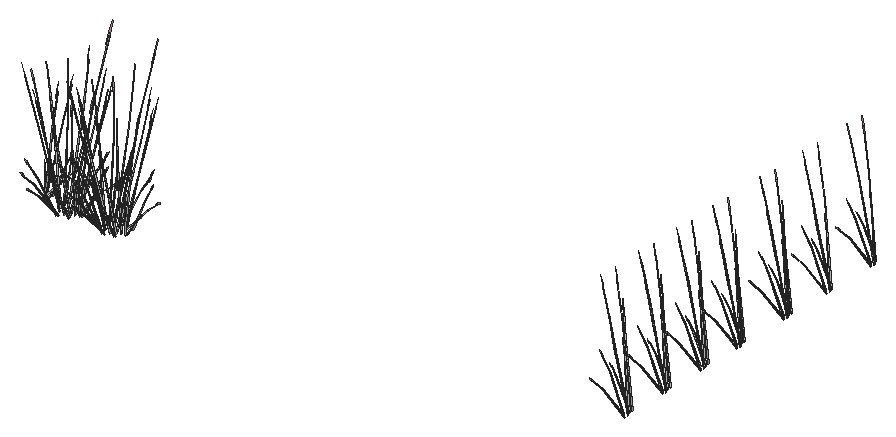
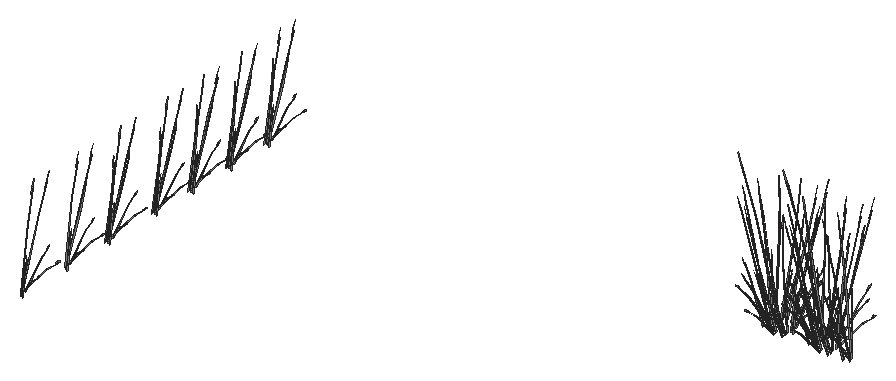
# SketchUp Ruby script. Lengths in inches.
U = 1.inch
M = Sketchup.active_model
def pt(a) = Geom::Point3d.new(a.map { |v| v * U })
def face(e, loops, mat)
  f = e.add_face(loops[0].map { |a| pt(a) })
  loops[1..].each { |l| e.add_face(l.map { |a| pt(a) }).erase! }
  f.material = f.back_material = mat if mat
  f
end
# faces: each face lists its corners as indices into pts; further lists are holes
def faces(e, pts, list, mat = nil) = list.each { |f| face(e, (f[0].is_a?(Array) ? f : [f]).map { |l| l.map { |i| pts[i] } }, mat) }
# xy, xz, yz: faces in a plane at the given z, y or x. An outline is a flat list of corners, or four numbers for a rectangle; further outlines are holes
def ring(l) = l.size == 4 ? [[l[0], l[1]], [l[2], l[1]], [l[2], l[3]], [l[0], l[3]]] : l.each_slice(2).to_a
def flat(e, list, mat, &to3) = list.each { |f| face(e, (f[0].is_a?(Array) ? f : [f]).map { |l| ring(l).map { |u, v| to3.(u, v) } }, mat) }
def xy(e, z, list, mat = nil) = flat(e, list, mat) { |x, y| [x, y, z] }
def xz(e, y, list, mat = nil) = flat(e, list, mat) { |x, z| [x, y, z] }
def yz(e, x, list, mat = nil) = flat(e, list, mat) { |y, z| [x, y, z] }
def lines(e, pts, list) = list.each { |a, b| e.add_line(pt(pts[a]), pt(pts[b])) }
# prism: a flat outline (further loops are holes) pulled along v
def prism(e, loops, v, mat = nil)
  f = face(e, loops, mat); d = Geom::Vector3d.new(v.map { |x| x * U })
  f.pushpull(f.normal.samedirection?(d) ? d.length : -d.length)
end
def box(e, o, s, mat = nil) = prism(e, [[o, [o[0] + s[0], o[1], o[2]], [o[0] + s[0], o[1] + s[1], o[2]], [o[0], o[1] + s[1], o[2]]]], [0, 0, s[2]], mat)
def at(x, y, z, deg = 0) = Geom::Transformation.translation(pt([x, y, z])) * Geom::Transformation.rotation(ORIGIN, Z_AXIS, deg.degrees)
def axes(o, x, y, z) = Geom::Transformation.new([*x, 0, *y, 0, *z, 0, *pt(o).to_a, 1])
def part(name) = M.definitions.add(name)
# library, detail: a bought-in or finely detailed component or shape, given as its bounding box
def library(name, o, s) = part(name).tap { |d| box(d.entities, o, s) }
def detail(e, o, s) = box(e.add_group.entities, o, s)
def put(e, d, t, mat = nil) = e.add_instance(d, t).tap { |i| i.material = mat if mat }
def group(e, t, mat = nil) = e.add_group.tap { |g| g.transformation = t; g.material = mat if mat }.entities
root = M.entities
M.materials.add("LightPink_Translucent").color = [144, 107, 117]
M.materials["LightPink_Translucent"].alpha = 0.75
M.materials.add("[_0053_Ivory_]").color = [200, 200, 200]
c1 = part("blade")
p = [[2.15,0.21,22],[0,0.17,0],[0.09,0.45,0],[2.18,0.31,22],[2.29,0.31,22],[0.38,0.45,0],
  [2.48,0.24,33],[2.49,0.24,33],[2.48,0.22,33]]
faces(c1.entities,p,[[0,1,2,3],[4,5,2,3],[6,3,4,7],[8,0,3,6]])
c2 = part("seeds")
p = [[0.3,-0.1,1.38],[-0.01,-0.03,1.59],[-0.01,-0.03,0.03],[0.14,-0.07,-0.07],[0.29,-0.03,3],[0.15,0.01,3.11]]
faces(c2.entities,p,[[0,1,2,3],[1,0,4,5]],"LightPink_Translucent")
c3 = part("blade with seeds")
put(c3.entities,c1,at(0,0,0))
put(c3.entities,c2,axes([2.4,0.25,30.99],[1.5799,-0.05474,1.17369],[-0.12525,1.92788,0.29478],[-0.07173,-0.02425,1.56792]))
put(root,c3,axes([467.79,99.63,131.37],[-0.13068,-0.00444,1.74944],[-0.41604,0.44388,-0.27667],[-0.22198,-0.0907,0.14031]),"[_0053_Ivory_]")
put(root,c3,axes([467.45,101.92,131.6875],[0.30559,0.56943,-0.1216],[-0.54237,0.27983,-0.67495],[-0.22856,0.07513,1.02557]),"[_0053_Ivory_]")
put(root,c3,axes([468.14,100.74,131.6875],[-0.03252,0.63953,-0.1216],[-0.61574,-0.01748,-0.67495],[-0.23714,-0.04442,1.02557]),"[_0053_Ivory_]")
put(root,c3,axes([462.59,102.55,131.36],[-0.07933,-0.00478,1.77383],[-0.32942,-0.51175,-0.16761],[0.13229,-0.16826,0.31391]),"[_0053_Ivory_]")
put(root,c3,axes([466.83,104.72,131.37],[-0.0151,0.12444,1.74944],[0.42844,0.43292,-0.27667],[-0.11216,0.20472,0.14031]),"[_0053_Ivory_]")
put(root,c3,axes([469.34,99.81,132.08],[-0.40534,0.60286,-0.13619],[-0.58702,-0.34732,-0.75594],[-0.20405,-0.17032,1.14864]),"[_0053_Ivory_]")
put(root,c3,axes([460.55,105.23,131.6875],[0.03252,-0.63953,-0.1216],[0.61574,0.01748,-0.67495],[0.23714,0.04442,1.02557]),"[_0053_Ivory_]")
put(root,c3,axes([461.23,104.05,131.6875],[-0.30559,-0.56943,-0.1216],[0.54237,-0.27983,-0.67495],[0.22856,-0.07513,1.02557]),"[_0053_Ivory_]")
put(root,c3,axes([467.47,103.28,131.6875],[0.56181,0.34675,-0.1216],[-0.32367,0.50216,-0.67495],[-0.15873,0.17455,1.02557]),"[_0053_Ivory_]")
put(root,c3,axes([461.08,104.85,131.37],[0.13029,-0.01064,1.74944],[0.35737,-0.48855,-0.27667],[0.23175,0.06449,0.14031]),"[_0053_Ivory_]")
put(root,c3,axes([469.18,98.37,131.36],[-0.01133,0.07538,1.77383],[-0.55883,0.27355,-0.16761],[-0.16445,-0.13983,0.31391]),"[_0053_Ivory_]")
put(root,c3,axes([462.45,105.74,131.36],[-0.05492,-0.05505,1.77383],[0.12013,-0.59013,-0.16761],[0.21632,-0.0377,0.31391]),"[_0053_Ivory_]")
put(root,c3,axes([466.78,105.99,131.36],[0.0689,-0.03797,1.77383],[0.5695,0.25254,-0.16761],[-0.01338,0.21027,0.31391]),"[_0053_Ivory_]")
put(root,c3,axes([462.89,103.16,131.37],[0.08428,-0.09579,1.74944],[-0.10787,-0.58756,-0.27667],[0.21147,-0.1114,0.14031]),"[_0053_Ivory_]")
put(root,c3,axes([469.82,98.66,131.37],[-0.0929,-0.08817,1.74944],[-0.61994,0.0559,-0.27667],[-0.09894,-0.21089,0.14031]),"[_0053_Ivory_]")
put(root,c3,axes([468.2,104.4375,132.05],[0.6675,0.03116,-0.13498],[-0.01824,0.58993,-0.74919],[-0.04637,0.2272,1.13838]),"[_0053_Ivory_]")
put(root,c3,axes([470.76,100.02,131.6875],[-0.59433,0.29278,-0.1216],[-0.29207,-0.51964,-0.67495],[-0.07842,-0.21898,1.02557]),"[_0053_Ivory_]")
put(root,c3,axes([469.29,106.26,131.37],[0.07699,0.10127,1.74944],[0.6213,0.03978,-0.27667],[0.06248,0.22333,0.14031]),"[_0053_Ivory_]")
put(root,c3,axes([469.43,105.09,131.6875],[0.59433,-0.29278,-0.1216],[0.29207,0.51964,-0.67495],[0.07842,0.21898,1.02557]),"[_0053_Ivory_]")
put(root,c3,axes([472.47,99.29,131.36],[-0.06168,0.04803,1.77383],[-0.60432,-0.16205,-0.16761],[-0.02188,-0.20961,0.31391]),"[_0053_Ivory_]")
put(root,c3,axes([472,100.68,131.6875],[-0.6675,-0.03116,-0.1216],[0.01824,-0.58993,-0.67495],[0.04637,-0.2272,1.02557]),"[_0053_Ivory_]")
put(root,c3,axes([471.26,101.9,131.13],[-0.52482,-0.32674,1.38283],[0.55416,-0.50872,0.59665],[0.16933,0.30658,1.33663]),"[_0053_Ivory_]")
put(root,c3,axes([470.375,105.52,131.36],[0.0018,-0.07613,1.77383],[0.52048,-0.3359,-0.16761],[0.18079,0.11989,0.31391]),"[_0053_Ivory_]")
put(root,c3,axes([472.6,99.74,131.37],[-0.00586,-0.12516,1.74944],[-0.49517,-0.36172,-0.27667],[0.07656,-0.21927,0.14031]),"[_0053_Ivory_]")
put(root,c3,axes([470.85,105.07,131.6875],[0.36191,-0.53827,-0.1216],[0.52412,0.3101,-0.67495],[0.18219,0.15207,1.02557]),"[_0053_Ivory_]")
put(root,c3,axes([472.72,101.84,131.6875],[-0.56181,-0.34675,-0.1216],[0.32367,-0.50216,-0.67495],[0.15873,-0.17455,1.02557]),"[_0053_Ivory_]")
put(root,c3,axes([474.11,101.69,131.36],[-0.07933,-0.00478,1.77383],[-0.32942,-0.51175,-0.16761],[0.13229,-0.16826,0.31391]),"[_0053_Ivory_]")
put(root,c3,axes([472.06,104.38,131.6875],[0.03252,-0.63953,-0.1216],[0.61574,0.01748,-0.67495],[0.23714,0.04442,1.02557]),"[_0053_Ivory_]")
put(root,c3,axes([472.75,103.19,131.6875],[-0.30559,-0.56943,-0.1216],[0.54237,-0.27983,-0.67495],[0.22856,-0.07513,1.02557]),"[_0053_Ivory_]")
put(root,c3,axes([481.3,102.28,131.37],[-0.09918,0.08165,1.74944],[0.00844,0.59653,-0.27667],[-0.22734,0.07758,0.14031]),"[_0053_Ivory_]")
put(root,c3,axes([472.59,103.99,131.37],[0.13029,-0.01064,1.74944],[0.35737,-0.48855,-0.27667],[0.23175,0.06449,0.14031]),"[_0053_Ivory_]")
put(root,c3,axes([480.2,102.88,131.36],[0.07751,0.01687,1.77383],[0.23978,0.55562,-0.16761],[-0.15867,0.14583,0.31391]),"[_0053_Ivory_]")
put(root,c3,axes([481.77,99.8,131.36],[0.04503,0.06276,1.77383],[-0.21706,0.56413,-0.16761],[-0.21983,0.00408,0.31391]),"[_0053_Ivory_]")
put(root,c3,axes([473.96,104.89,131.36],[-0.05492,-0.05505,1.77383],[0.12013,-0.59013,-0.16761],[0.21632,-0.0377,0.31391]),"[_0053_Ivory_]")
put(root,c3,axes([482.28,99.42,131.37],[-0.13068,-0.00444,1.74944],[-0.41604,0.44388,-0.27667],[-0.22198,-0.0907,0.14031]),"[_0053_Ivory_]")
put(root,c3,axes([481.94,101.71,131.6875],[0.30559,0.56943,-0.1216],[-0.54237,0.27983,-0.67495],[-0.22856,0.07513,1.02557]),"[_0053_Ivory_]")
put(root,c3,axes([482.63,100.53,131.6875],[-0.03252,0.63953,-0.1216],[-0.61574,-0.01748,-0.67495],[-0.23714,-0.04442,1.02557]),"[_0053_Ivory_]")
put(root,c3,axes([474.41,102.3,131.37],[0.08428,-0.09579,1.74944],[-0.10787,-0.58756,-0.27667],[0.21147,-0.1114,0.14031]),"[_0053_Ivory_]")
put(root,c3,axes([481.32,104.51,131.37],[-0.0151,0.12444,1.74944],[0.42844,0.43292,-0.27667],[-0.11216,0.20472,0.14031]),"[_0053_Ivory_]")
put(root,c3,axes([483.83,99.6,132.08],[-0.40534,0.60286,-0.13619],[-0.58702,-0.34732,-0.75594],[-0.20405,-0.17032,1.14864]),"[_0053_Ivory_]")
put(root,c3,axes([481.97,103.07,131.6875],[0.56181,0.34675,-0.1216],[-0.32367,0.50216,-0.67495],[-0.15873,0.17455,1.02557]),"[_0053_Ivory_]")
put(root,c3,axes([483.67,98.16,131.36],[-0.01133,0.07538,1.77383],[-0.55883,0.27355,-0.16761],[-0.16445,-0.13983,0.31391]),"[_0053_Ivory_]")
put(root,c3,axes([481.27,105.78,131.36],[0.0689,-0.03797,1.77383],[0.5695,0.25254,-0.16761],[-0.01338,0.21027,0.31391]),"[_0053_Ivory_]")
put(root,c3,axes([484.31,98.45,131.37],[-0.0929,-0.08817,1.74944],[-0.61994,0.0559,-0.27667],[-0.09894,-0.21089,0.14031]),"[_0053_Ivory_]")
put(root,c3,axes([482.69,104.23,132.05],[0.6675,0.03116,-0.13498],[-0.01824,0.58993,-0.74919],[-0.04637,0.2272,1.13838]),"[_0053_Ivory_]")
put(root,c3,axes([485.25,99.8125,131.6875],[-0.59433,0.29278,-0.1216],[-0.29207,-0.51964,-0.67495],[-0.07842,-0.21898,1.02557]),"[_0053_Ivory_]")
put(root,c3,axes([483.79,106.05,131.37],[0.07699,0.10127,1.74944],[0.6213,0.03978,-0.27667],[0.06248,0.22333,0.14031]),"[_0053_Ivory_]")
put(root,c3,axes([483.93,104.89,131.6875],[0.59433,-0.29278,-0.1216],[0.29207,0.51964,-0.67495],[0.07842,0.21898,1.02557]),"[_0053_Ivory_]")
put(root,c3,axes([486.96,99.08,131.36],[-0.06168,0.04803,1.77383],[-0.60432,-0.16205,-0.16761],[-0.02188,-0.20961,0.31391]),"[_0053_Ivory_]")
put(root,c3,axes([486.49,100.47,131.6875],[-0.6675,-0.03116,-0.1216],[0.01824,-0.58993,-0.67495],[0.04637,-0.2272,1.02557]),"[_0053_Ivory_]")
put(root,c3,axes([485.75,101.6875,131.13],[-0.52482,-0.32674,1.38283],[0.55416,-0.50872,0.59665],[0.16933,0.30658,1.33663]),"[_0053_Ivory_]")
put(root,c3,axes([484.86,105.31,131.36],[0.0018,-0.07613,1.77383],[0.52048,-0.3359,-0.16761],[0.18079,0.11989,0.31391]),"[_0053_Ivory_]")
put(root,c3,axes([487.09,99.53,131.37],[-0.00586,-0.12516,1.74944],[-0.49517,-0.36172,-0.27667],[0.07656,-0.21927,0.14031]),"[_0053_Ivory_]")
put(root,c3,axes([485.34,104.86,131.6875],[0.36191,-0.53827,-0.1216],[0.52412,0.3101,-0.67495],[0.18219,0.15207,1.02557]),"[_0053_Ivory_]")
put(root,c3,axes([487.21,101.63,131.6875],[-0.56181,-0.34675,-0.1216],[0.32367,-0.50216,-0.67495],[0.15873,-0.17455,1.02557]),"[_0053_Ivory_]")
put(root,c3,axes([488.6,101.48,131.36],[-0.07933,-0.00478,1.77383],[-0.32942,-0.51175,-0.16761],[0.13229,-0.16826,0.31391]),"[_0053_Ivory_]")
put(root,c3,axes([486.55,104.17,131.6875],[0.03252,-0.63953,-0.1216],[0.61574,0.01748,-0.67495],[0.23714,0.04442,1.02557]),"[_0053_Ivory_]")
put(root,c3,axes([487.24,102.98,131.6875],[-0.30559,-0.56943,-0.1216],[0.54237,-0.27983,-0.67495],[0.22856,-0.07513,1.02557]),"[_0053_Ivory_]")
put(root,c3,axes([487.09,103.78,131.37],[0.13029,-0.01064,1.74944],[0.35737,-0.48855,-0.27667],[0.23175,0.06449,0.14031]),"[_0053_Ivory_]")
put(root,c3,axes([488.45,104.68,131.36],[-0.05492,-0.05505,1.77383],[0.12013,-0.59013,-0.16761],[0.21632,-0.0377,0.31391]),"[_0053_Ivory_]")
put(root,c3,axes([488.9,102.09,131.37],[0.08428,-0.09579,1.74944],[-0.10787,-0.58756,-0.27667],[0.21147,-0.1114,0.14031]),"[_0053_Ivory_]")
put(root,c3,axes([640.54,109.39,131.37],[-0.09918,0.08165,1.74944],[0.00844,0.59653,-0.27667],[-0.22734,0.07758,0.14031]),"[_0053_Ivory_]")
put(root,c3,axes([640.54,124.46,131.37],[-0.09918,0.08165,1.74944],[0.00844,0.59653,-0.27667],[-0.22734,0.07758,0.14031]),"[_0053_Ivory_]")
put(root,c3,axes([640.54,139.37,131.37],[-0.09918,0.08165,1.74944],[0.00844,0.59653,-0.27667],[-0.22734,0.07758,0.14031]),"[_0053_Ivory_]")
put(root,c3,axes([640.54,153.65,131.37],[-0.09918,0.08165,1.74944],[0.00844,0.59653,-0.27667],[-0.22734,0.07758,0.14031]),"[_0053_Ivory_]")
put(root,c3,axes([640.54,172.13,131.37],[-0.09918,0.08165,1.74944],[0.00844,0.59653,-0.27667],[-0.22734,0.07758,0.14031]),"[_0053_Ivory_]")
put(root,c3,axes([640.54,188.89,131.37],[-0.09918,0.08165,1.74944],[0.00844,0.59653,-0.27667],[-0.22734,0.07758,0.14031]),"[_0053_Ivory_]")
put(root,c3,axes([640.54,206.48,131.37],[-0.09918,0.08165,1.74944],[0.00844,0.59653,-0.27667],[-0.22734,0.07758,0.14031]),"[_0053_Ivory_]")
put(root,c3,axes([639.4375,109.99,131.36],[0.07751,0.01687,1.77383],[0.23978,0.55562,-0.16761],[-0.15867,0.14583,0.31391]),"[_0053_Ivory_]")
put(root,c3,axes([639.4375,125.06,131.36],[0.07751,0.01687,1.77383],[0.23978,0.55562,-0.16761],[-0.15867,0.14583,0.31391]),"[_0053_Ivory_]")
put(root,c3,axes([639.4375,139.97,131.36],[0.07751,0.01687,1.77383],[0.23978,0.55562,-0.16761],[-0.15867,0.14583,0.31391]),"[_0053_Ivory_]")
put(root,c3,axes([639.4375,154.25,131.36],[0.07751,0.01687,1.77383],[0.23978,0.55562,-0.16761],[-0.15867,0.14583,0.31391]),"[_0053_Ivory_]")
put(root,c3,axes([639.4375,172.73,131.36],[0.07751,0.01687,1.77383],[0.23978,0.55562,-0.16761],[-0.15867,0.14583,0.31391]),"[_0053_Ivory_]")
put(root,c3,axes([639.4375,189.49,131.36],[0.07751,0.01687,1.77383],[0.23978,0.55562,-0.16761],[-0.15867,0.14583,0.31391]),"[_0053_Ivory_]")
put(root,c3,axes([639.4375,207.08,131.36],[0.07751,0.01687,1.77383],[0.23978,0.55562,-0.16761],[-0.15867,0.14583,0.31391]),"[_0053_Ivory_]")
put(root,c3,axes([641.01,106.91,131.36],[0.04503,0.06276,1.77383],[-0.21706,0.56413,-0.16761],[-0.21983,0.00408,0.31391]),"[_0053_Ivory_]")
put(root,c3,axes([641.01,121.97,131.36],[0.04503,0.06276,1.77383],[-0.21706,0.56413,-0.16761],[-0.21983,0.00408,0.31391]),"[_0053_Ivory_]")
put(root,c3,axes([641.01,136.89,131.36],[0.04503,0.06276,1.77383],[-0.21706,0.56413,-0.16761],[-0.21983,0.00408,0.31391]),"[_0053_Ivory_]")
put(root,c3,axes([641.01,151.16,131.36],[0.04503,0.06276,1.77383],[-0.21706,0.56413,-0.16761],[-0.21983,0.00408,0.31391]),"[_0053_Ivory_]")
put(root,c3,axes([641.01,169.65,131.36],[0.04503,0.06276,1.77383],[-0.21706,0.56413,-0.16761],[-0.21983,0.00408,0.31391]),"[_0053_Ivory_]")
put(root,c3,axes([641.01,186.41,131.36],[0.04503,0.06276,1.77383],[-0.21706,0.56413,-0.16761],[-0.21983,0.00408,0.31391]),"[_0053_Ivory_]")
put(root,c3,axes([641.01,204,131.36],[0.04503,0.06276,1.77383],[-0.21706,0.56413,-0.16761],[-0.21983,0.00408,0.31391]),"[_0053_Ivory_]")
put(root,c3,axes([641.51,106.53,131.37],[-0.13068,-0.00444,1.74944],[-0.41604,0.44388,-0.27667],[-0.22198,-0.0907,0.14031]),"[_0053_Ivory_]")
put(root,c3,axes([641.51,121.6,131.37],[-0.13068,-0.00444,1.74944],[-0.41604,0.44388,-0.27667],[-0.22198,-0.0907,0.14031]),"[_0053_Ivory_]")
put(root,c3,axes([641.51,136.51,131.37],[-0.13068,-0.00444,1.74944],[-0.41604,0.44388,-0.27667],[-0.22198,-0.0907,0.14031]),"[_0053_Ivory_]")
put(root,c3,axes([641.51,150.79,131.37],[-0.13068,-0.00444,1.74944],[-0.41604,0.44388,-0.27667],[-0.22198,-0.0907,0.14031]),"[_0053_Ivory_]")
put(root,c3,axes([641.51,169.27,131.37],[-0.13068,-0.00444,1.74944],[-0.41604,0.44388,-0.27667],[-0.22198,-0.0907,0.14031]),"[_0053_Ivory_]")
put(root,c3,axes([641.51,186.03,131.37],[-0.13068,-0.00444,1.74944],[-0.41604,0.44388,-0.27667],[-0.22198,-0.0907,0.14031]),"[_0053_Ivory_]")
put(root,c3,axes([641.51,203.62,131.37],[-0.13068,-0.00444,1.74944],[-0.41604,0.44388,-0.27667],[-0.22198,-0.0907,0.14031]),"[_0053_Ivory_]")
put(root,c3,axes([641.18,108.82,131.6875],[0.30559,0.56943,-0.1216],[-0.54237,0.27983,-0.67495],[-0.22856,0.07513,1.02557]),"[_0053_Ivory_]")
put(root,c3,axes([641.18,123.89,131.6875],[0.30559,0.56943,-0.1216],[-0.54237,0.27983,-0.67495],[-0.22856,0.07513,1.02557]),"[_0053_Ivory_]")
put(root,c3,axes([641.18,138.8,131.6875],[0.30559,0.56943,-0.1216],[-0.54237,0.27983,-0.67495],[-0.22856,0.07513,1.02557]),"[_0053_Ivory_]")
put(root,c3,axes([641.18,153.08,131.6875],[0.30559,0.56943,-0.1216],[-0.54237,0.27983,-0.67495],[-0.22856,0.07513,1.02557]),"[_0053_Ivory_]")
put(root,c3,axes([641.18,171.5625,131.6875],[0.30559,0.56943,-0.1216],[-0.54237,0.27983,-0.67495],[-0.22856,0.07513,1.02557]),"[_0053_Ivory_]")
put(root,c3,axes([641.18,188.32,131.6875],[0.30559,0.56943,-0.1216],[-0.54237,0.27983,-0.67495],[-0.22856,0.07513,1.02557]),"[_0053_Ivory_]")
put(root,c3,axes([641.18,205.91,131.6875],[0.30559,0.56943,-0.1216],[-0.54237,0.27983,-0.67495],[-0.22856,0.07513,1.02557]),"[_0053_Ivory_]")
put(root,c3,axes([641.87,107.64,131.6875],[-0.03252,0.63953,-0.1216],[-0.61574,-0.01748,-0.67495],[-0.23714,-0.04442,1.02557]),"[_0053_Ivory_]")
put(root,c3,axes([641.87,122.7,131.6875],[-0.03252,0.63953,-0.1216],[-0.61574,-0.01748,-0.67495],[-0.23714,-0.04442,1.02557]),"[_0053_Ivory_]")
put(root,c3,axes([641.87,137.62,131.6875],[-0.03252,0.63953,-0.1216],[-0.61574,-0.01748,-0.67495],[-0.23714,-0.04442,1.02557]),"[_0053_Ivory_]")
put(root,c3,axes([641.87,151.9,131.6875],[-0.03252,0.63953,-0.1216],[-0.61574,-0.01748,-0.67495],[-0.23714,-0.04442,1.02557]),"[_0053_Ivory_]")
put(root,c3,axes([641.87,170.38,131.6875],[-0.03252,0.63953,-0.1216],[-0.61574,-0.01748,-0.67495],[-0.23714,-0.04442,1.02557]),"[_0053_Ivory_]")
put(root,c3,axes([641.87,187.14,131.6875],[-0.03252,0.63953,-0.1216],[-0.61574,-0.01748,-0.67495],[-0.23714,-0.04442,1.02557]),"[_0053_Ivory_]")
put(root,c3,axes([641.87,204.73,131.6875],[-0.03252,0.63953,-0.1216],[-0.61574,-0.01748,-0.67495],[-0.23714,-0.04442,1.02557]),"[_0053_Ivory_]")
put(root,c3,axes([640.93,108.83,131.38],[-0.22307,-0.42878,0.0643],[0.40677,-0.20987,0.50621],[-0.17931,0.04141,0.77189]),"[_0053_Ivory_]")
put(root,c3,axes([640.93,123.9,131.38],[-0.22307,-0.42878,0.0643],[0.40677,-0.20987,0.50621],[-0.17931,0.04141,0.77189]),"[_0053_Ivory_]")
put(root,c3,axes([640.93,138.82,131.38],[-0.22307,-0.42878,0.0643],[0.40677,-0.20987,0.50621],[-0.17931,0.04141,0.77189]),"[_0053_Ivory_]")
put(root,c3,axes([640.93,153.09,131.38],[-0.22307,-0.42878,0.0643],[0.40677,-0.20987,0.50621],[-0.17931,0.04141,0.77189]),"[_0053_Ivory_]")
put(root,c3,axes([640.93,171.57,131.38],[-0.22307,-0.42878,0.0643],[0.40677,-0.20987,0.50621],[-0.17931,0.04141,0.77189]),"[_0053_Ivory_]")
put(root,c3,axes([640.93,188.33,131.38],[-0.22307,-0.42878,0.0643],[0.40677,-0.20987,0.50621],[-0.17931,0.04141,0.77189]),"[_0053_Ivory_]")
put(root,c3,axes([641,110.3,131.38],[-0.41695,-0.26447,0.0643],[0.24275,-0.37662,0.50621],[-0.13368,0.12176,0.77189]),"[_0053_Ivory_]")
put(root,c3,axes([641,125.37,131.38],[-0.41695,-0.26447,0.0643],[0.24275,-0.37662,0.50621],[-0.13368,0.12176,0.77189]),"[_0053_Ivory_]")
put(root,c3,axes([641,140.28,131.38],[-0.41695,-0.26447,0.0643],[0.24275,-0.37662,0.50621],[-0.13368,0.12176,0.77189]),"[_0053_Ivory_]")
put(root,c3,axes([641,154.56,131.38],[-0.41695,-0.26447,0.0643],[0.24275,-0.37662,0.50621],[-0.13368,0.12176,0.77189]),"[_0053_Ivory_]")
put(root,c3,axes([641,173.04,131.38],[-0.41695,-0.26447,0.0643],[0.24275,-0.37662,0.50621],[-0.13368,0.12176,0.77189]),"[_0053_Ivory_]")
